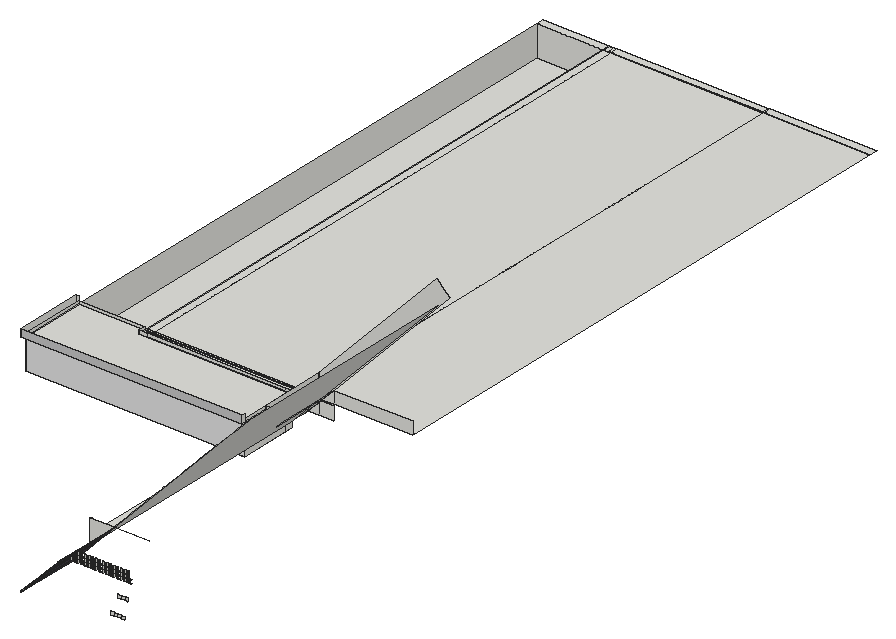
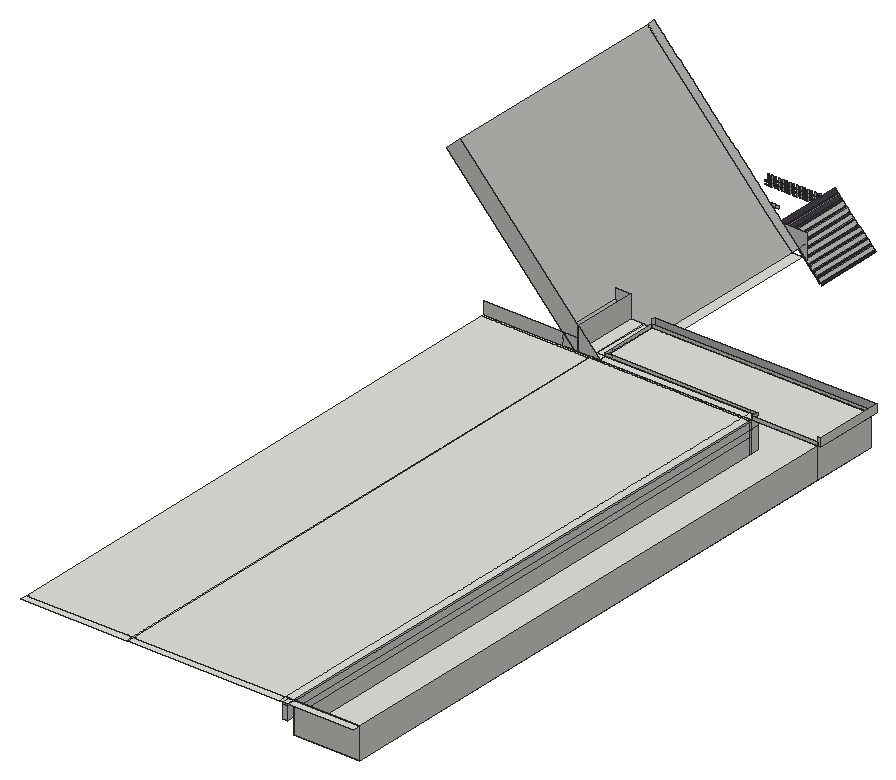
# SketchUp Ruby script. Lengths in inches.
U = 1.inch
M = Sketchup.active_model
def pt(a) = Geom::Point3d.new(a.map { |v| v * U })
def face(e, loops, mat)
  f = e.add_face(loops[0].map { |a| pt(a) })
  loops[1..].each { |l| e.add_face(l.map { |a| pt(a) }).erase! }
  f.material = f.back_material = mat if mat
  f
end
# faces: each face lists its corners as indices into pts; further lists are holes
def faces(e, pts, list, mat = nil) = list.each { |f| face(e, (f[0].is_a?(Array) ? f : [f]).map { |l| l.map { |i| pts[i] } }, mat) }
# xy, xz, yz: faces in a plane at the given z, y or x. An outline is a flat list of corners, or four numbers for a rectangle; further outlines are holes
def ring(l) = l.size == 4 ? [[l[0], l[1]], [l[2], l[1]], [l[2], l[3]], [l[0], l[3]]] : l.each_slice(2).to_a
def flat(e, list, mat, &to3) = list.each { |f| face(e, (f[0].is_a?(Array) ? f : [f]).map { |l| ring(l).map { |u, v| to3.(u, v) } }, mat) }
def xy(e, z, list, mat = nil) = flat(e, list, mat) { |x, y| [x, y, z] }
def xz(e, y, list, mat = nil) = flat(e, list, mat) { |x, z| [x, y, z] }
def yz(e, x, list, mat = nil) = flat(e, list, mat) { |y, z| [x, y, z] }
def lines(e, pts, list) = list.each { |a, b| e.add_line(pt(pts[a]), pt(pts[b])) }
# prism: a flat outline (further loops are holes) pulled along v
def prism(e, loops, v, mat = nil)
  f = face(e, loops, mat); d = Geom::Vector3d.new(v.map { |x| x * U })
  f.pushpull(f.normal.samedirection?(d) ? d.length : -d.length)
end
def box(e, o, s, mat = nil) = prism(e, [[o, [o[0] + s[0], o[1], o[2]], [o[0] + s[0], o[1] + s[1], o[2]], [o[0], o[1] + s[1], o[2]]]], [0, 0, s[2]], mat)
def at(x, y, z, deg = 0) = Geom::Transformation.translation(pt([x, y, z])) * Geom::Transformation.rotation(ORIGIN, Z_AXIS, deg.degrees)
def axes(o, x, y, z) = Geom::Transformation.new([*x, 0, *y, 0, *z, 0, *pt(o).to_a, 1])
def part(name) = M.definitions.add(name)
# library, detail: a bought-in or finely detailed component or shape, given as its bounding box
def library(name, o, s) = part(name).tap { |d| box(d.entities, o, s) }
def detail(e, o, s) = box(e.add_group.entities, o, s)
def put(e, d, t, mat = nil) = e.add_instance(d, t).tap { |i| i.material = mat if mat }
def group(e, t, mat = nil) = e.add_group.tap { |g| g.transformation = t; g.material = mat if mat }.entities
root = M.entities
M.materials.add("[Color M01]").color = [226, 226, 226]
M.materials.add("[Color M02]").color = [198, 198, 198]
M.materials.add("[Color M06]").color = [79, 71, 84]
xy(root,315.25,[[252.64,678.64,252.64,1195.68,306.21,1195.68,306.21,726.125,429.58,726.125,429.58,678.64]])
xy(root,326.08,[[428,528.48,436.5,719.2],[428,719.2,436.5,719.59]])
xy(root,333.125,[[306.21,726.125,310.02,732.2],[306.21,732.2,310.02,734.4375],[306.21,734.4375,310.02,1195.68]])
xy(root,333.71,[[444.85,480.14,447.16,480.77],[447.76,480.14,450.07,480.77],[450.67,480.14,452.98,480.77],[453.58,480.14,455.89,480.77],[456.49,480.14,458.81,480.77],
  [459.41,480.14,461.72,480.77],[462.32,480.14,464.63,480.77],[465.23,480.14,467.54,480.77],[468.14,480.14,470.45,480.77],[471.05,480.14,473.37,480.77],
  [473.97,480.14,476.28,480.77],[476.88,480.14,479.19,480.77],[479.79,480.14,482.1,480.77],[482.7,480.14,485.02,480.77],[485.61,480.14,487.93,480.77],
  [488.53,480.14,490.84,480.77],[491.4375,480.14,493.75,480.77],[494.35,480.14,496.66,480.77]])
xy(root,336.02,[[446.91,480.14,447.16,480.77],[447.76,480.14,450.07,480.77],[450.67,480.14,452.98,480.77],[453.58,480.14,455.89,480.77],[456.49,480.14,458.81,480.77],
  [459.41,480.14,461.72,480.77],[462.32,480.14,464.63,480.77],[465.23,480.14,467.54,480.77],[468.14,480.14,470.45,480.77],[471.05,480.14,473.37,480.77],
  [473.97,480.14,476.28,480.77],[476.88,480.14,479.19,480.77],[479.79,480.14,482.1,480.77],[482.7,480.14,485.02,480.77],[485.61,480.14,487.93,480.77],
  [488.53,480.14,490.84,480.77],[491.4375,480.14,493.75,480.77],[494.35,480.14,496.66,480.77]])
xy(root,336.52,[[447.76,480.14,450.07,480.77],[450.67,480.14,452.98,480.77],[453.58,480.14,455.89,480.77],[456.49,480.14,458.81,480.77],[459.41,480.14,461.72,480.77],
  [462.32,480.14,464.63,480.77],[465.23,480.14,467.54,480.77],[468.14,480.14,470.45,480.77],[471.05,480.14,473.37,480.77],[473.97,480.14,476.28,480.77],
  [476.88,480.14,479.19,480.77],[479.79,480.14,482.1,480.77],[482.7,480.14,485.02,480.77],[485.61,480.14,487.93,480.77],[488.53,480.14,490.84,480.77],
  [491.4375,480.14,493.75,480.77],[494.35,480.14,496.66,480.77]])
xy(root,338.84,[[449.55,480.14,450.07,480.77],[450.67,480.14,452.98,480.77],[453.58,480.14,455.89,480.77],[456.49,480.14,458.81,480.77],[459.41,480.14,461.72,480.77],
  [462.32,480.14,464.63,480.77],[465.23,480.14,467.54,480.77],[468.14,480.14,470.45,480.77],[471.05,480.14,473.37,480.77],[473.97,480.14,476.28,480.77],
  [476.88,480.14,479.19,480.77],[479.79,480.14,482.1,480.77],[482.7,480.14,485.02,480.77],[485.61,480.14,487.93,480.77],[488.53,480.14,490.84,480.77],
  [491.4375,480.14,493.75,480.77]])
xy(root,339.34,[[450.67,480.14,452.98,480.77],[453.58,480.14,455.89,480.77],[456.49,480.14,458.81,480.77],[459.41,480.14,461.72,480.77],[462.32,480.14,464.63,480.77],
  [465.23,480.14,467.54,480.77],[468.14,480.14,470.45,480.77],[471.05,480.14,473.37,480.77],[473.97,480.14,476.28,480.77],[476.88,480.14,479.19,480.77],
  [479.79,480.14,482.1,480.77],[482.7,480.14,485.02,480.77],[485.61,480.14,487.93,480.77],[488.53,480.14,490.84,480.77],[491.4375,480.14,493.75,480.77]])
xy(root,340.125,[[250.08,676.08,252.64,678.64],[252.64,676.08,429.58,678.64],[250.08,678.64,252.64,732.2],[252.64,678.64,252.64,732.2,306.21,732.2,306.21,726.125,429.58,726.125,429.58,678.64],[429.58,678.64,435.78,726.125],
  [435.78,678.64,436.5,726.125],[436.5,678.64,446.875,726.125],[446.875,678.64,449.72,726.125],[306.21,726.125,312.28,732.2],[312.28,726.125,435.78,732.2],
  [436.5,726.125,446.875,732.2],[446.875,726.125,449.72,732.2],[306.21,732.2,312.28,734.4375],[312.28,732.2,435.78,732.2,435.78,732.32,312.41,732.32,312.41,734.4375,312.28,734.4375],[435.78,732.2,436.5,734.4375],
  [436.5,732.2,522.625,734.4375],[312.41,732.32,435.78,734.4375],[306.21,734.4375,312.28,1195.68],[312.28,734.4375,312.41,1195.68],[312.41,734.4375,435.78,1195.68],
  [435.78,734.4375,436.5,1195.68],[436.5,734.4375,522.625,1195.68],[252.64,1195.68,306.21,1195.8],[306.21,1195.68,310.02,1195.8],[310.02,1195.68,312.28,1195.8],
  [312.28,1195.68,435.78,1195.8],[435.78,1195.68,436.5,1195.8],[436.5,1195.68,522.625,1195.8],[252.64,1195.8,306.21,1201.875],[306.21,1195.8,310.02,1201.875],
  [310.02,1195.8,312.28,1201.875],[312.28,1195.8,435.78,1201.875],[435.78,1195.8,436.5,1201.875],[436.5,1195.8,522.625,1201.875]])
xz(root,480.64,[[479.76,305.35,482.07,307.67],[482.67,305.35,484.99,307.67],[485.59,305.35,487.9,307.67],[488.5,305.35,490.81,307.67]])
xz(root,480.7,[[485.61,319.65,487.93,321.96],[488.53,319.65,490.84,321.96],[491.4375,319.65,493.75,321.96]])
xz(root,521.5625,[[419.07,306.65,418.61,307.08,421.04,309.65,421.49,309.22],[418.61,307.08,418.39,307.29,420.81,309.87,421.04,309.65],[422.37,310.16,421.91,310.59,424.33,313.16,424.79,312.73],[425.67,313.66,425.21,314.09,427.63,316.66,428.09,316.23],[428.96,317.17,428.51,317.59,429.58,318.73,429.58,317.82],
  [429.58,317.82,430.04,318.3,429.58,318.73],[430.04,318.3,431.39,319.74,430.93,320.17,429.58,318.73],[429.58,318.73,430.93,320.17,431.81,321.1,434.23,323.67,435.11,324.6,436.5,326.08,437.53,327.17,438.41,328.11,440.83,330.68,441.7,331.61,444.125,334.18,445,335.11,447.42,337.6875,448.3,338.62,449.72,340.125,429.58,340.125],[432.26,320.67,434.68,323.24,434.23,323.67,431.81,321.1],[435.5625,324.17,435.11,324.6,436.5,326.08,436.5,325.17],
  [436.5,325.17,436.96,325.65,436.5,326.08],[436.96,325.65,437.98,326.75,437.53,327.17,436.5,326.08],[438.86,327.68,441.28,330.25,440.83,330.68,438.41,328.11],[442.16,331.18,444.58,333.75,444.125,334.18,441.7,331.61],[445.46,334.6875,447.88,337.26,447.42,337.6875,445,335.11],
  [448.76,338.19,450.17,339.7,449.72,340.125,448.3,338.62],[450.17,339.7,450.58,340.125,449.72,340.125],[449.72,340.125,450.58,340.125,451.18,340.76,450.72,341.19]])
xz(root,676.08,[[250.08,340.125,429.58,346.3125]],"[Color M02]")
xz(root,678.64,[[252.64,340.125,429.58,342.6875],[446.875,340.125,449.72,340.125,459.19,350.1875,459.19,358.5,446.875,358.5]])
xz(root,678.64,[[252.64,315.25,429.58,340.125]],"[Color M01]")
xz(root,726.125,[[306.21,315.25,310.02,333.125],[310.02,315.25,312.28,315.25,312.28,340.125,306.21,340.125,306.21,333.125,310.02,333.125],[312.28,315.25,424.39,340.125],[424.39,315.25,429.58,340.125],[306.21,340.125,312.28,342.6875],
  [312.28,340.125,424.39,342.6875],[424.39,340.125,429.58,342.6875]])
xz(root,731.75,[[436.5,326.08,425.82,336.13,429.58,340.125,446.15,357.73,446.875,357.04,446.875,358.5,542.88,460.49,550.41,453.39,553.56,450.4375,459.19,350.1875,449.72,340.125]])
xz(root,732.2,[[436.5,326.08,436.5,328,438.31,328],[306.21,328,312.28,338.875],[312.28,328,436.5,338.875],[436.5,328,436.5,338.875,446.875,338.875,446.875,337.11,438.31,328],[438.31,328,446.875,328,446.875,337.11],
  [446.875,328,459.19,328,459.19,338.875,448.54,338.875,446.875,337.11],[446.875,337.11,446.875,338.875,448.54,338.875],[306.21,338.875,312.28,340.125],[312.28,338.875,436.5,340.125],[436.5,338.875,446.875,340.125],
  [446.875,338.875,446.875,340.125,449.72,340.125,448.54,338.875],[448.54,338.875,459.19,338.875,459.19,340.125,449.72,340.125],[250.08,340.125,252.64,346.3125],[252.64,340.125,306.21,342.6875],[446.875,340.125,446.875,350.1875,459.19,350.1875,449.72,340.125],
  [449.72,340.125,459.19,350.1875,459.19,340.125],[459.19,340.125,522.625,350.1875]])
xz(root,1195.68,[[252.64,315.25,306.21,340.125],[306.21,333.125,310.02,340.125]])
xz(root,1201.875,[[306.21,328,310.02,338.875],[306.21,338.875,310.02,340.125]])
yz(root,250.08,[[676.08,340.125,732.2,346.3125]])
yz(root,252.64,[[678.64,315.25,732.2,340.125],[732.2,315.25,1195.68,340.125],[678.64,340.125,732.2,342.6875]])
yz(root,306.21,[[726.125,315.25,732.2,333.125],[732.2,315.25,734.4375,328],[734.4375,315.25,1195.68,328],[732.2,328,734.4375,333.125],[734.4375,328,1195.68,333.125],
  [1195.68,328,1201.875,338.875],[726.125,333.125,732.2,340.125],[732.2,333.125,734.4375,338.875],[734.4375,333.125,1195.68,338.875],[732.2,338.875,734.4375,340.125],
  [734.4375,338.875,1195.68,340.125],[1195.68,338.875,1201.875,340.125],[726.125,340.125,732.2,342.6875]])
yz(root,429.58,[[678.64,315.25,719.59,340.125],[719.59,315.25,726.125,340.125],[676.08,340.125,678.64,346.3125],[678.64,340.125,719.59,342.6875],[719.59,340.125,726.125,342.6875]])
yz(root,436.5,[[726.125,326.08,732.2,340.125]])
yz(root,444.85,[[480.14,333.71,480.77,333.82]])
yz(root,446.875,[[678.64,340.125,731.75,358.5],[731.75,340.125,732.2,358.5]])
yz(root,447.16,[[480.14,333.71,480.77,336.02]])
yz(root,447.76,[[480.14,333.71,480.77,336.02],[480.14,336.52,480.77,336.93]])
yz(root,450.07,[[480.14,333.71,480.77,336.02],[480.14,336.52,480.77,338.84]])
yz(root,450.67,[[480.14,333.71,480.77,336.02],[480.14,336.52,480.77,338.84],[480.14,339.34,480.77,340.04]])
yz(root,452.98,[[480.14,333.71,480.77,336.02],[480.14,336.52,480.77,338.84],[480.14,339.34,480.77,341.65]])
yz(root,453.58,[[480.14,333.71,480.77,336.02],[480.14,336.52,480.77,338.84],[480.14,339.34,480.77,341.65]])
yz(root,455.89,[[480.14,333.71,480.77,336.02],[480.14,336.52,480.77,338.84],[480.14,339.34,480.77,341.65]])
yz(root,456.49,[[480.14,333.71,480.77,336.02],[480.14,336.52,480.77,338.84],[480.14,339.34,480.77,341.65]])
yz(root,458.81,[[480.14,333.71,480.77,336.02],[480.14,336.52,480.77,338.84],[480.14,339.34,480.77,341.65]])
yz(root,459.41,[[480.14,333.71,480.77,336.02],[480.14,336.52,480.77,338.84],[480.14,339.34,480.77,341.65]])
yz(root,461.72,[[480.14,333.71,480.77,336.02],[480.14,336.52,480.77,338.84],[480.14,339.34,480.77,341.65]])
yz(root,462.32,[[480.14,333.71,480.77,336.02],[480.14,336.52,480.77,338.84],[480.14,339.34,480.77,341.65]])
yz(root,464.63,[[480.14,333.71,480.77,336.02],[480.14,336.52,480.77,338.84],[480.14,339.34,480.77,341.65]])
yz(root,465.23,[[480.14,333.71,480.77,336.02],[480.14,336.52,480.77,338.84],[480.14,339.34,480.77,341.65]])
yz(root,467.54,[[480.14,333.71,480.77,336.02],[480.14,336.52,480.77,338.84],[480.14,339.34,480.77,341.65]])
yz(root,468.14,[[480.14,333.71,480.77,336.02],[480.14,336.52,480.77,338.84],[480.14,339.34,480.77,341.65]])
yz(root,470.45,[[480.14,333.71,480.77,336.02],[480.14,336.52,480.77,338.84],[480.14,339.34,480.77,341.65]])
yz(root,471.05,[[480.14,333.71,480.77,336.02],[480.14,336.52,480.77,338.84],[480.14,339.34,480.77,341.65]])
yz(root,473.37,[[480.14,333.71,480.77,336.02],[480.14,336.52,480.77,338.84],[480.14,339.34,480.77,341.65]])
yz(root,473.97,[[480.14,333.71,480.77,336.02],[480.14,336.52,480.77,338.84],[480.14,339.34,480.77,341.65]])
yz(root,476.28,[[480.14,333.71,480.77,336.02],[480.14,336.52,480.77,338.84],[480.14,339.34,480.77,341.65]])
yz(root,476.88,[[480.14,333.71,480.77,336.02],[480.14,336.52,480.77,338.84],[480.14,339.34,480.77,341.65]])
yz(root,479.19,[[480.14,333.71,480.77,336.02],[480.14,336.52,480.77,338.84],[480.14,339.34,480.77,341.65]])
yz(root,479.79,[[480.14,333.71,480.77,336.02],[480.14,336.52,480.77,338.84],[480.14,339.34,480.77,341.65]])
yz(root,482.1,[[480.14,333.71,480.77,336.02],[480.14,336.52,480.77,338.84],[480.14,339.34,480.77,341.65]])
yz(root,482.7,[[480.14,333.71,480.77,336.02],[480.14,336.52,480.77,338.84],[480.14,339.34,480.77,341.65]])
yz(root,485.02,[[480.14,333.71,480.77,336.02],[480.14,336.52,480.77,338.84],[480.14,339.34,480.77,341.65]])
yz(root,485.61,[[480.14,333.71,480.77,336.02],[480.14,336.52,480.77,338.84],[480.14,339.34,480.77,341.65]])
yz(root,487.93,[[480.14,333.71,480.77,336.02],[480.14,336.52,480.77,338.84],[480.14,339.34,480.77,341.65]])
yz(root,488.53,[[480.14,333.71,480.77,336.02],[480.14,336.52,480.77,338.84],[480.14,339.34,480.77,341.65]])
yz(root,490.84,[[480.14,333.71,480.77,336.02],[480.14,336.52,480.77,338.84],[480.14,339.34,480.77,341.65]])
yz(root,491.4375,[[480.14,333.71,480.77,336.02],[480.14,336.52,480.77,338.84],[480.14,339.34,480.77,341.65]])
yz(root,493.75,[[480.14,333.71,480.77,336.02],[480.14,336.52,480.77,338.84],[480.14,339.34,480.77,341.65]])
yz(root,494.35,[[480.14,336.52,480.77,338.84],[480.14,339.34,480.77,341.65]])
p = [[417.74,521.5625,306.15],[417.74,467.1875,306.15],[418.19,467.1875,305.72],[418.19,521.5625,305.72],[417.51,521.5625,306.36],[417.51,467.1875,306.36],
  [418.61,521.5625,307.08],[418.61,467.1875,307.08],[419.07,521.5625,306.65],[419.07,467.1875,306.65],[421.49,521.5625,309.22],[421.49,467.1875,309.22],
  [418.39,467.1875,307.29],[418.39,521.5625,307.29],[421.04,521.5625,309.65],[421.04,467.1875,309.65],[420.81,521.5625,309.87],[420.81,467.1875,309.87],
  [421.91,521.5625,310.59],[421.91,467.1875,310.59],[422.37,521.5625,310.16],[422.37,467.1875,310.16],[424.79,521.5625,312.73],[424.79,467.1875,312.73],
  [424.33,521.5625,313.16],[424.33,467.1875,313.16],[425.21,521.5625,314.09],[425.21,467.1875,314.09],[425.67,521.5625,313.66],[425.67,467.1875,313.66],
  [428.09,521.5625,316.23],[428.09,467.1875,316.23],[427.63,521.5625,316.66],[427.63,467.1875,316.66],[428.51,521.5625,317.59],[428.51,467.1875,317.59],
  [428.96,521.5625,317.17],[428.96,467.1875,317.17],[430.04,521.5625,318.3],[431.39,521.5625,319.74],[431.39,467.1875,319.74],[429.58,521.5625,317.82],
  [430.93,521.5625,320.17],[429.58,521.5625,318.73],[430.93,467.1875,320.17],[431.81,521.5625,321.1],[431.81,467.1875,321.1],[432.26,521.5625,320.67],
  [432.26,467.1875,320.67],[434.68,521.5625,323.24],[434.68,467.1875,323.24],[434.23,521.5625,323.67],[434.23,467.1875,323.67],[435.11,521.5625,324.6],
  [435.11,467.1875,324.6],[435.5625,521.5625,324.17],[435.5625,467.1875,324.17],[436.96,521.5625,325.65],[437.98,521.5625,326.75],[437.98,467.1875,326.75],
  [436.5,521.5625,325.17],[437.53,521.5625,327.17],[436.5,521.5625,326.08],[437.53,467.1875,327.17],[436.5,528.48,326.08],[553.56,528.48,450.4375],
  [553.56,521.5625,450.4375],[553.25,521.5625,450.11],[552.98,521.5625,449.82],[550.56,521.5625,447.25],[549.68,521.5625,446.32],[547.26,521.5625,443.75],
  [546.38,521.5625,442.8125],[543.96,521.5625,440.24],[543.08,521.5625,439.31],[540.66,521.5625,436.74],[539.78,521.5625,435.81],[537.36,521.5625,433.23],
  [536.48,521.5625,432.3],[534.0625,521.5625,429.73],[533.19,521.5625,428.8],[530.76,521.5625,426.23],[529.89,521.5625,425.29],[527.47,521.5625,422.72],
  [526.59,521.5625,421.79],[524.17,521.5625,419.22],[523.29,521.5625,418.28],[520.87,521.5625,415.71],[519.99,521.5625,414.78],[517.57,521.5625,412.21],
  [516.69,521.5625,411.28],[514.27,521.5625,408.7],[513.39,521.5625,407.77],[510.97,521.5625,405.2],[510.1,521.5625,404.27],[507.67,521.5625,401.7],
  [506.8,521.5625,400.76],[504.375,521.5625,398.19],[503.5,521.5625,397.26],[501.08,521.5625,394.6875],[500.2,521.5625,393.75],[497.78,521.5625,391.18],
  [496.9,521.5625,390.25],[494.48,521.5625,387.68],[493.6,521.5625,386.75],[491.18,521.5625,384.17],[490.3,521.5625,383.24],[487.88,521.5625,380.67],
  [487.01,521.5625,379.74],[484.58,521.5625,377.17],[483.71,521.5625,376.23],[481.29,521.5625,373.66],[480.41,521.5625,372.73],[477.99,521.5625,370.16],
  [477.11,521.5625,369.23],[474.6875,521.5625,366.65],[473.8125,521.5625,365.72],[471.39,521.5625,363.15],[470.51,521.5625,362.22],[468.09,521.5625,359.64],
  [467.21,521.5625,358.71],[464.79,521.5625,356.14],[463.92,521.5625,355.21],[461.49,521.5625,352.64],[460.62,521.5625,351.7],[458.2,521.5625,349.13],
  [457.32,521.5625,348.2],[454.9,521.5625,345.63],[454.02,521.5625,344.7],[451.6,521.5625,342.125],[450.72,521.5625,341.19],[449.72,521.5625,340.125],
  [448.3,521.5625,338.62],[447.42,521.5625,337.6875],[445,521.5625,335.11],[444.125,521.5625,334.18],[441.7,521.5625,331.61],[440.83,521.5625,330.68],
  [438.41,521.5625,328.11],[436.5,719.59,326.08],[449.72,719.59,340.125],[449.72,678.64,340.125],[459.19,678.64,350.1875],[459.19,719.59,350.1875],
  [553.56,719.59,450.4375],[436.5,719.2,326.08],[425.82,719.2,336.13],[425.82,731.75,336.13],[436.5,731.75,326.08],[436.5,726.125,326.08],
  [449.72,726.125,340.125],[449.72,731.75,340.125],[449.72,732.2,340.125],[448.54,732.2,338.875],[446.875,732.2,337.11],[438.31,732.2,328],
  [436.5,732.2,326.08],[438.41,467.1875,328.11],[438.86,521.5625,327.68],[438.86,467.1875,327.68],[441.28,521.5625,330.25],[441.28,467.1875,330.25],
  [440.83,467.1875,330.68],[441.7,467.1875,331.61],[442.16,521.5625,331.18],[442.16,467.1875,331.18],[444.58,521.5625,333.75],[444.58,467.1875,333.75],
  [444.125,467.1875,334.18],[446.91,480.14,336.02],[444.85,480.14,333.82],[444.85,480.77,333.82],[446.91,480.77,336.02],[445,467.1875,335.11],
  [445.46,521.5625,334.6875],[445.46,467.1875,334.6875],[447.88,521.5625,337.26],[447.88,467.1875,337.26],[449.55,480.14,338.84],[447.76,480.14,336.93],
  [447.76,480.77,336.93],[449.55,480.77,338.84],[447.42,467.1875,337.6875],[448.3,467.1875,338.62],[448.76,521.5625,338.19],[448.76,467.1875,338.19],
  [450.58,521.5625,340.125],[451.18,521.5625,340.76],[451.18,467.1875,340.76],[450.17,521.5625,339.7],[452.18,480.14,341.65],[450.67,480.14,340.04],
  [450.67,480.77,340.04],[452.18,480.77,341.65],[459.19,731.75,350.1875],[459.19,732.2,350.1875],[425.82,528.48,336.13],[429.58,726.125,340.125],
  [429.58,731.75,340.125],[478.55,521.5625,340.125]]
faces(root,p,[[0,1,2,3],[1,0,4,5],[6,7,12,13],[14,6,7,15],[16,13,12,17],[14,15,11,10],[15,14,16,17],[24,18,19,25],
  [24,25,23,22],[27,26,28,29],[32,26,27,33],[32,33,31,30],[35,34,36,37],[42,43,34,35,44],[42,44,40,39],[46,45,47,48],
  [51,45,46,52],[51,52,50,49],[54,53,55,56],[61,62,53,54,63],[64,65,66,67,68,69,70,71,72,73,74,75,76,77,78,79,80,81,82,83,84,85,86,87,88,89,90,91,92,93,94,95,96,97,98,99,100,101,102,103,104,105,106,107,108,109,110,111,112,113,114,115,116,117,118,119,120,121,122,123,124,125,126,127,128,129,130,131,132,133,134,135,136,137,138,61,62],[139,140,141,142,143,144,65,64,145],[139,145,146,147,148,149],[139,140,150,151,148,149],
  [148,151,152,153,154,155,156],[61,63,59,58],[157,138,158,159],[137,138,157,162],[137,162,161,160],[163,136,164,165],[135,136,163,168],[135,168,167,166],
  [169,170,171,172],[173,134,174,175],[178,179,180,181],[133,182,177,176],[183,132,184,185],[190,191,192,193],[140,143,142,141],[140,143,194,151,150],
  [194,151,152,195]])
faces(root,p,[[0,6,7,1],[7,6,8,9],[8,10,11,9],[14,18,19,15],[19,18,20,21],[20,22,23,21],[24,26,27,25],[28,30,31,29],
  [32,34,35,33],[38,39,40,37,36,41],[42,45,46,44],[47,49,50,48],[51,53,54,52],[57,58,59,56,55,60],[61,138,157,63],[158,160,161,159],
  [137,136,163,162],[164,166,167,165],[135,134,173,168],[174,176,177,175],[133,132,183,182],[186,187,188,185,184,189]],"[Color M06]")
lines(root,p,[[64,196],[197,198],[199,186]])
